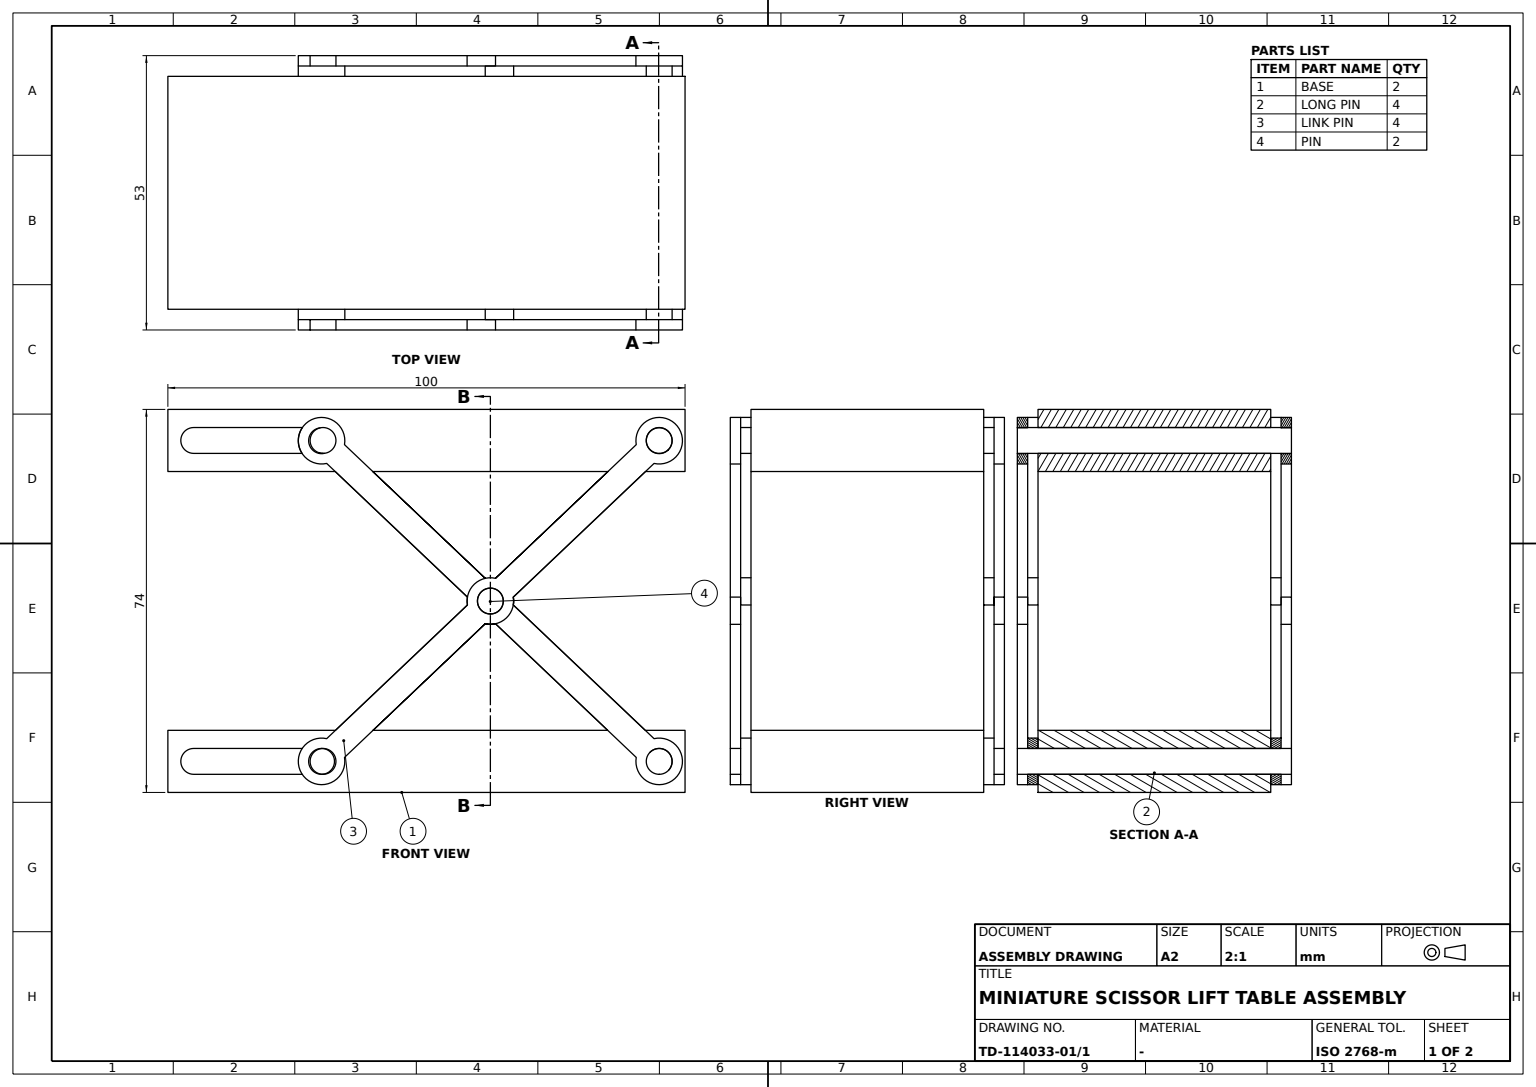
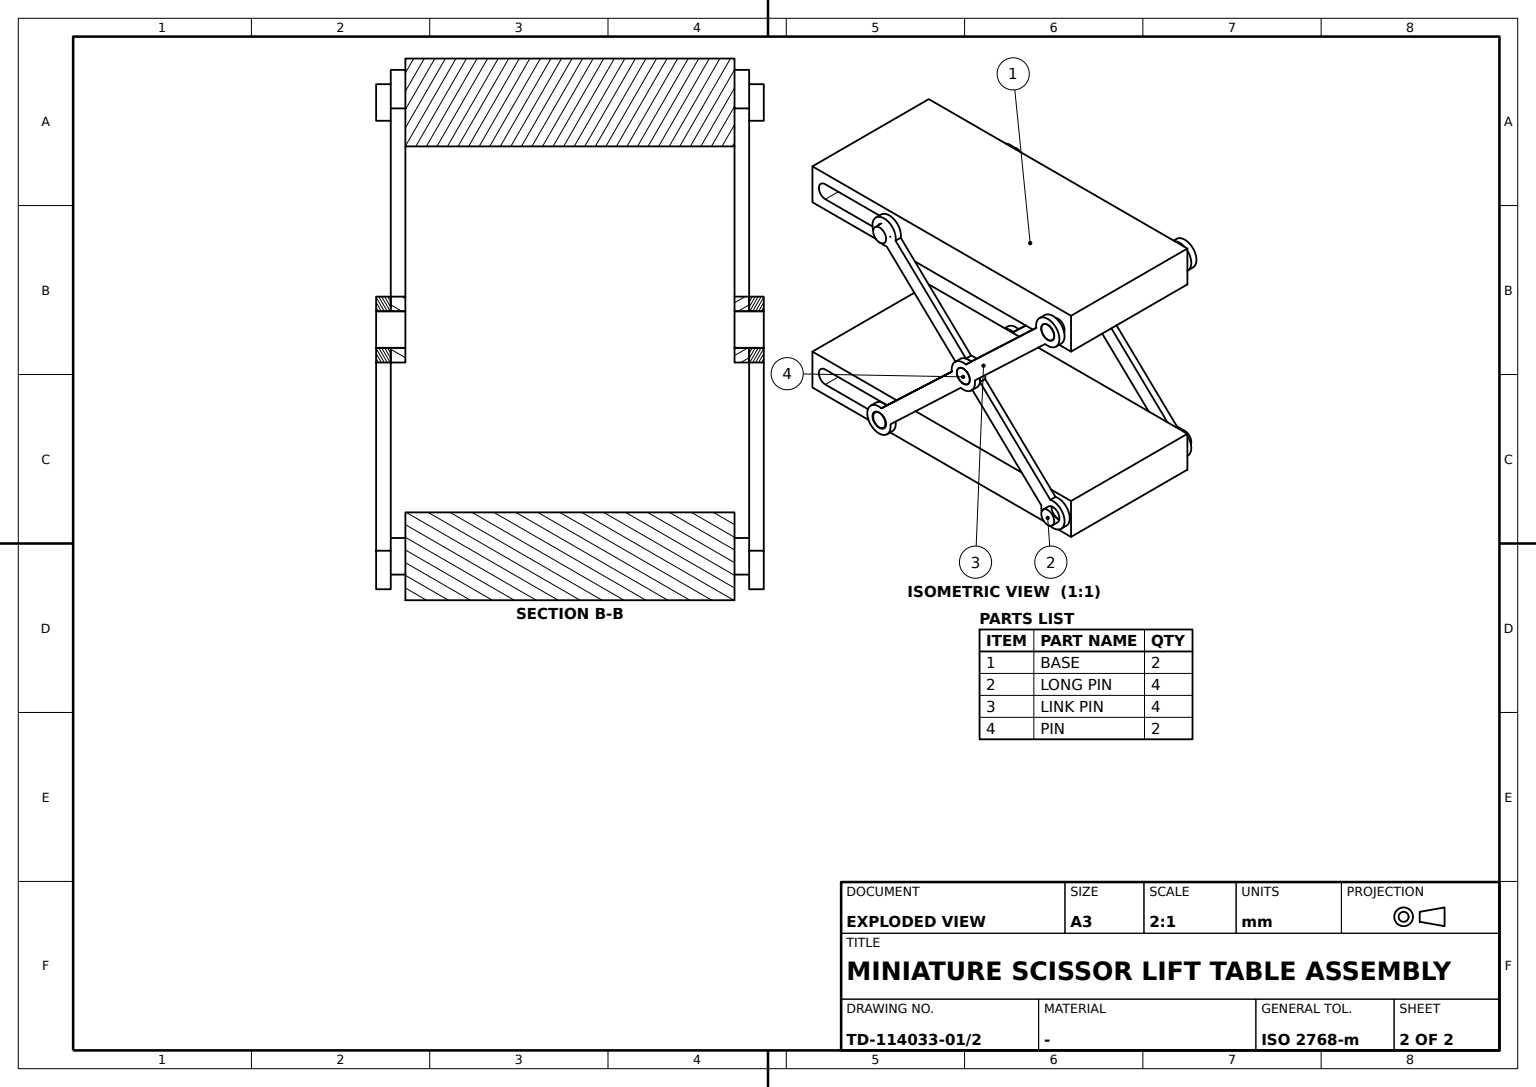
ISO-10303-21;
HEADER;
FILE_DESCRIPTION((''),'2;1');
FILE_NAME('','',(''),(''),'','','');
FILE_SCHEMA(('AUTOMOTIVE_DESIGN'));
ENDSEC;
DATA;
#11=LINE('',#845,#47);
#12=LINE('',#849,#48);
#13=LINE('',#853,#49);
#14=LINE('',#857,#50);
#15=LINE('',#865,#51);
#16=LINE('',#870,#52);
#17=LINE('',#874,#53);
#18=LINE('',#878,#54);
#19=LINE('',#885,#55);
#20=LINE('',#886,#56);
#21=LINE('',#888,#57);
#22=LINE('',#890,#58);
#23=LINE('',#892,#59);
#24=LINE('',#894,#60);
#25=LINE('',#896,#61);
#26=LINE('',#898,#62);
#27=LINE('',#917,#63);
#28=LINE('',#921,#64);
#29=LINE('',#928,#65);
#30=LINE('',#931,#66);
#31=LINE('',#933,#67);
#32=LINE('',#935,#68);
#33=LINE('',#937,#69);
#34=LINE('',#940,#70);
#35=LINE('',#941,#71);
#36=LINE('',#943,#72);
#37=LINE('',#946,#73);
#38=LINE('',#947,#74);
#39=LINE('',#949,#75);
#40=LINE('',#950,#76);
#41=LINE('',#952,#77);
#42=LINE('',#954,#78);
#43=LINE('',#956,#79);
#44=LINE('',#958,#80);
#45=LINE('',#964,#81);
#46=LINE('',#966,#82);
#47=VECTOR('',#681,1000.);
#48=VECTOR('',#684,1000.);
#49=VECTOR('',#687,1000.);
#50=VECTOR('',#690,1000.);
#51=VECTOR('',#699,1000.);
#52=VECTOR('',#702,1000.);
#53=VECTOR('',#705,1000.);
#54=VECTOR('',#708,1000.);
#55=VECTOR('',#719,1000.);
#56=VECTOR('',#720,1000.);
#57=VECTOR('',#723,1000.);
#58=VECTOR('',#726,1000.);
#59=VECTOR('',#729,1000.);
#60=VECTOR('',#732,1000.);
#61=VECTOR('',#735,1000.);
#62=VECTOR('',#738,1000.);
#63=VECTOR('',#767,1000.);
#64=VECTOR('',#770,1000.);
#65=VECTOR('',#779,1000.);
#66=VECTOR('',#780,1000.);
#67=VECTOR('',#781,1000.);
#68=VECTOR('',#782,1000.);
#69=VECTOR('',#785,1000.);
#70=VECTOR('',#786,1000.);
#71=VECTOR('',#787,1000.);
#72=VECTOR('',#790,1000.);
#73=VECTOR('',#791,1000.);
#74=VECTOR('',#792,1000.);
#75=VECTOR('',#795,1000.);
#76=VECTOR('',#796,1000.);
#77=VECTOR('',#799,1000.);
#78=VECTOR('',#800,1000.);
#79=VECTOR('',#801,1000.);
#80=VECTOR('',#804,1000.);
#81=VECTOR('',#811,1000.);
#82=VECTOR('',#814,1000.);
#83=CONTEXT_DEPENDENT_SHAPE_REPRESENTATION(#107,#988);
#84=CONTEXT_DEPENDENT_SHAPE_REPRESENTATION(#108,#989);
#85=CONTEXT_DEPENDENT_SHAPE_REPRESENTATION(#109,#991);
#86=CONTEXT_DEPENDENT_SHAPE_REPRESENTATION(#110,#992);
#87=CONTEXT_DEPENDENT_SHAPE_REPRESENTATION(#111,#993);
#88=CONTEXT_DEPENDENT_SHAPE_REPRESENTATION(#112,#994);
#89=CONTEXT_DEPENDENT_SHAPE_REPRESENTATION(#113,#996);
#90=CONTEXT_DEPENDENT_SHAPE_REPRESENTATION(#114,#997);
#91=CONTEXT_DEPENDENT_SHAPE_REPRESENTATION(#115,#999);
#92=CONTEXT_DEPENDENT_SHAPE_REPRESENTATION(#116,#1000);
#93=CONTEXT_DEPENDENT_SHAPE_REPRESENTATION(#117,#1001);
#94=CONTEXT_DEPENDENT_SHAPE_REPRESENTATION(#118,#1002);
#95=NEXT_ASSEMBLY_USAGE_OCCURRENCE('pin','pin','pin',#1003,#1004,'');
#96=NEXT_ASSEMBLY_USAGE_OCCURRENCE('pin','pin','pin',#1003,#1004,'');
#97=NEXT_ASSEMBLY_USAGE_OCCURRENCE('link pin','link pin','link pin',#1003,#1005,'');
#98=NEXT_ASSEMBLY_USAGE_OCCURRENCE('link pin','link pin','link pin',#1003,#1005,'');
#99=NEXT_ASSEMBLY_USAGE_OCCURRENCE('link pin','link pin','link pin',#1003,#1005,'');
#100=NEXT_ASSEMBLY_USAGE_OCCURRENCE('link pin','link pin','link pin',#1003,#1005,'');
#101=NEXT_ASSEMBLY_USAGE_OCCURRENCE('long pin','long pin','long pin',#1003,#1006,'');
#102=NEXT_ASSEMBLY_USAGE_OCCURRENCE('long pin','long pin','long pin',#1003,#1006,'');
#103=NEXT_ASSEMBLY_USAGE_OCCURRENCE('base','base','base',#1003,#1007,'');
#104=NEXT_ASSEMBLY_USAGE_OCCURRENCE('long pin','long pin','long pin',#1003,#1006,'');
#105=NEXT_ASSEMBLY_USAGE_OCCURRENCE('long pin','long pin','long pin',#1003,#1006,'');
#106=NEXT_ASSEMBLY_USAGE_OCCURRENCE('base','base','base',#1003,#1007,'');
#107=(REPRESENTATION_RELATIONSHIP(' ',' ',#584,#583)REPRESENTATION_RELATIONSHIP_WITH_TRANSFORMATION(#119)SHAPE_REPRESENTATION_RELATIONSHIP());
#108=(REPRESENTATION_RELATIONSHIP(' ',' ',#584,#583)REPRESENTATION_RELATIONSHIP_WITH_TRANSFORMATION(#120)SHAPE_REPRESENTATION_RELATIONSHIP());
#109=(REPRESENTATION_RELATIONSHIP(' ',' ',#585,#583)REPRESENTATION_RELATIONSHIP_WITH_TRANSFORMATION(#121)SHAPE_REPRESENTATION_RELATIONSHIP());
#110=(REPRESENTATION_RELATIONSHIP(' ',' ',#585,#583)REPRESENTATION_RELATIONSHIP_WITH_TRANSFORMATION(#122)SHAPE_REPRESENTATION_RELATIONSHIP());
#111=(REPRESENTATION_RELATIONSHIP(' ',' ',#585,#583)REPRESENTATION_RELATIONSHIP_WITH_TRANSFORMATION(#123)SHAPE_REPRESENTATION_RELATIONSHIP());
#112=(REPRESENTATION_RELATIONSHIP(' ',' ',#585,#583)REPRESENTATION_RELATIONSHIP_WITH_TRANSFORMATION(#124)SHAPE_REPRESENTATION_RELATIONSHIP());
#113=(REPRESENTATION_RELATIONSHIP(' ',' ',#586,#583)REPRESENTATION_RELATIONSHIP_WITH_TRANSFORMATION(#125)SHAPE_REPRESENTATION_RELATIONSHIP());
#114=(REPRESENTATION_RELATIONSHIP(' ',' ',#586,#583)REPRESENTATION_RELATIONSHIP_WITH_TRANSFORMATION(#126)SHAPE_REPRESENTATION_RELATIONSHIP());
#115=(REPRESENTATION_RELATIONSHIP(' ',' ',#587,#583)REPRESENTATION_RELATIONSHIP_WITH_TRANSFORMATION(#127)SHAPE_REPRESENTATION_RELATIONSHIP());
#116=(REPRESENTATION_RELATIONSHIP(' ',' ',#586,#583)REPRESENTATION_RELATIONSHIP_WITH_TRANSFORMATION(#128)SHAPE_REPRESENTATION_RELATIONSHIP());
#117=(REPRESENTATION_RELATIONSHIP(' ',' ',#586,#583)REPRESENTATION_RELATIONSHIP_WITH_TRANSFORMATION(#129)SHAPE_REPRESENTATION_RELATIONSHIP());
#118=(REPRESENTATION_RELATIONSHIP(' ',' ',#587,#583)REPRESENTATION_RELATIONSHIP_WITH_TRANSFORMATION(#130)SHAPE_REPRESENTATION_RELATIONSHIP());
#119=ITEM_DEFINED_TRANSFORMATION(' ',' ',#588,#594);
#120=ITEM_DEFINED_TRANSFORMATION(' ',' ',#588,#595);
#121=ITEM_DEFINED_TRANSFORMATION(' ',' ',#588,#623);
#122=ITEM_DEFINED_TRANSFORMATION(' ',' ',#588,#624);
#123=ITEM_DEFINED_TRANSFORMATION(' ',' ',#588,#625);
#124=ITEM_DEFINED_TRANSFORMATION(' ',' ',#588,#626);
#125=ITEM_DEFINED_TRANSFORMATION(' ',' ',#588,#632);
#126=ITEM_DEFINED_TRANSFORMATION(' ',' ',#588,#633);
#127=ITEM_DEFINED_TRANSFORMATION(' ',' ',#588,#651);
#128=ITEM_DEFINED_TRANSFORMATION(' ',' ',#588,#652);
#129=ITEM_DEFINED_TRANSFORMATION(' ',' ',#588,#653);
#130=ITEM_DEFINED_TRANSFORMATION(' ',' ',#588,#654);
#131=SHAPE_REPRESENTATION_RELATIONSHIP('','',#584,#135);
#132=SHAPE_REPRESENTATION_RELATIONSHIP('','',#585,#136);
#133=SHAPE_REPRESENTATION_RELATIONSHIP('','',#586,#137);
#134=SHAPE_REPRESENTATION_RELATIONSHIP('','',#587,#138);
#135=ADVANCED_BREP_SHAPE_REPRESENTATION('',(#574),#974);
#136=ADVANCED_BREP_SHAPE_REPRESENTATION('',(#575),#975);
#137=ADVANCED_BREP_SHAPE_REPRESENTATION('',(#576),#976);
#138=ADVANCED_BREP_SHAPE_REPRESENTATION('',(#577),#977);
#139=CYLINDRICAL_SURFACE('',#593,2.5);
#140=CYLINDRICAL_SURFACE('',#612,2.5);
#141=CYLINDRICAL_SURFACE('',#613,2.5);
#142=CYLINDRICAL_SURFACE('',#614,2.5);
#143=CYLINDRICAL_SURFACE('',#616,4.5);
#144=CYLINDRICAL_SURFACE('',#618,4.5);
#145=CYLINDRICAL_SURFACE('',#620,4.5);
#146=CYLINDRICAL_SURFACE('',#622,4.5);
#147=CYLINDRICAL_SURFACE('',#631,2.5);
#148=CYLINDRICAL_SURFACE('',#634,2.5);
#149=CYLINDRICAL_SURFACE('',#637,2.5);
#150=CYLINDRICAL_SURFACE('',#649,2.5);
#151=ORIENTED_EDGE('',*,*,#271,.T.);
#152=ORIENTED_EDGE('',*,*,#272,.F.);
#153=ORIENTED_EDGE('',*,*,#271,.F.);
#154=ORIENTED_EDGE('',*,*,#272,.T.);
#155=ORIENTED_EDGE('',*,*,#273,.F.);
#156=ORIENTED_EDGE('',*,*,#274,.F.);
#157=ORIENTED_EDGE('',*,*,#275,.F.);
#158=ORIENTED_EDGE('',*,*,#276,.T.);
#159=ORIENTED_EDGE('',*,*,#277,.T.);
#160=ORIENTED_EDGE('',*,*,#278,.T.);
#161=ORIENTED_EDGE('',*,*,#279,.T.);
#162=ORIENTED_EDGE('',*,*,#280,.T.);
#163=ORIENTED_EDGE('',*,*,#281,.F.);
#164=ORIENTED_EDGE('',*,*,#282,.T.);
#165=ORIENTED_EDGE('',*,*,#283,.F.);
#166=ORIENTED_EDGE('',*,*,#284,.T.);
#167=ORIENTED_EDGE('',*,*,#285,.T.);
#168=ORIENTED_EDGE('',*,*,#286,.T.);
#169=ORIENTED_EDGE('',*,*,#287,.T.);
#170=ORIENTED_EDGE('',*,*,#288,.F.);
#171=ORIENTED_EDGE('',*,*,#289,.T.);
#172=ORIENTED_EDGE('',*,*,#290,.F.);
#173=ORIENTED_EDGE('',*,*,#291,.F.);
#174=ORIENTED_EDGE('',*,*,#292,.F.);
#175=ORIENTED_EDGE('',*,*,#293,.F.);
#176=ORIENTED_EDGE('',*,*,#294,.F.);
#177=ORIENTED_EDGE('',*,*,#273,.T.);
#178=ORIENTED_EDGE('',*,*,#284,.F.);
#179=ORIENTED_EDGE('',*,*,#274,.T.);
#180=ORIENTED_EDGE('',*,*,#285,.F.);
#181=ORIENTED_EDGE('',*,*,#275,.T.);
#182=ORIENTED_EDGE('',*,*,#286,.F.);
#183=ORIENTED_EDGE('',*,*,#295,.F.);
#184=ORIENTED_EDGE('',*,*,#287,.F.);
#185=ORIENTED_EDGE('',*,*,#296,.T.);
#186=ORIENTED_EDGE('',*,*,#283,.T.);
#187=ORIENTED_EDGE('',*,*,#297,.F.);
#188=ORIENTED_EDGE('',*,*,#288,.T.);
#189=ORIENTED_EDGE('',*,*,#295,.T.);
#190=ORIENTED_EDGE('',*,*,#282,.F.);
#191=ORIENTED_EDGE('',*,*,#298,.F.);
#192=ORIENTED_EDGE('',*,*,#289,.F.);
#193=ORIENTED_EDGE('',*,*,#297,.T.);
#194=ORIENTED_EDGE('',*,*,#281,.T.);
#195=ORIENTED_EDGE('',*,*,#299,.F.);
#196=ORIENTED_EDGE('',*,*,#290,.T.);
#197=ORIENTED_EDGE('',*,*,#298,.T.);
#198=ORIENTED_EDGE('',*,*,#280,.F.);
#199=ORIENTED_EDGE('',*,*,#300,.F.);
#200=ORIENTED_EDGE('',*,*,#291,.T.);
#201=ORIENTED_EDGE('',*,*,#299,.T.);
#202=ORIENTED_EDGE('',*,*,#279,.F.);
#203=ORIENTED_EDGE('',*,*,#301,.F.);
#204=ORIENTED_EDGE('',*,*,#292,.T.);
#205=ORIENTED_EDGE('',*,*,#300,.T.);
#206=ORIENTED_EDGE('',*,*,#278,.F.);
#207=ORIENTED_EDGE('',*,*,#302,.F.);
#208=ORIENTED_EDGE('',*,*,#293,.T.);
#209=ORIENTED_EDGE('',*,*,#301,.T.);
#210=ORIENTED_EDGE('',*,*,#277,.F.);
#211=ORIENTED_EDGE('',*,*,#296,.F.);
#212=ORIENTED_EDGE('',*,*,#294,.T.);
#213=ORIENTED_EDGE('',*,*,#302,.T.);
#214=ORIENTED_EDGE('',*,*,#276,.F.);
#215=ORIENTED_EDGE('',*,*,#303,.T.);
#216=ORIENTED_EDGE('',*,*,#304,.F.);
#217=ORIENTED_EDGE('',*,*,#303,.F.);
#218=ORIENTED_EDGE('',*,*,#304,.T.);
#219=ORIENTED_EDGE('',*,*,#305,.F.);
#220=ORIENTED_EDGE('',*,*,#306,.F.);
#221=ORIENTED_EDGE('',*,*,#307,.T.);
#222=ORIENTED_EDGE('',*,*,#308,.T.);
#223=ORIENTED_EDGE('',*,*,#309,.F.);
#224=ORIENTED_EDGE('',*,*,#310,.T.);
#225=ORIENTED_EDGE('',*,*,#311,.F.);
#226=ORIENTED_EDGE('',*,*,#312,.F.);
#227=ORIENTED_EDGE('',*,*,#313,.T.);
#228=ORIENTED_EDGE('',*,*,#314,.T.);
#229=ORIENTED_EDGE('',*,*,#315,.F.);
#230=ORIENTED_EDGE('',*,*,#316,.F.);
#231=ORIENTED_EDGE('',*,*,#311,.T.);
#232=ORIENTED_EDGE('',*,*,#317,.T.);
#233=ORIENTED_EDGE('',*,*,#318,.F.);
#234=ORIENTED_EDGE('',*,*,#319,.F.);
#235=ORIENTED_EDGE('',*,*,#315,.T.);
#236=ORIENTED_EDGE('',*,*,#320,.T.);
#237=ORIENTED_EDGE('',*,*,#313,.F.);
#238=ORIENTED_EDGE('',*,*,#321,.F.);
#239=ORIENTED_EDGE('',*,*,#318,.T.);
#240=ORIENTED_EDGE('',*,*,#322,.T.);
#241=ORIENTED_EDGE('',*,*,#323,.T.);
#242=ORIENTED_EDGE('',*,*,#324,.F.);
#243=ORIENTED_EDGE('',*,*,#325,.F.);
#244=ORIENTED_EDGE('',*,*,#306,.T.);
#245=ORIENTED_EDGE('',*,*,#309,.T.);
#246=ORIENTED_EDGE('',*,*,#326,.F.);
#247=ORIENTED_EDGE('',*,*,#327,.T.);
#248=ORIENTED_EDGE('',*,*,#323,.F.);
#249=ORIENTED_EDGE('',*,*,#305,.T.);
#250=ORIENTED_EDGE('',*,*,#312,.T.);
#251=ORIENTED_EDGE('',*,*,#316,.T.);
#252=ORIENTED_EDGE('',*,*,#319,.T.);
#253=ORIENTED_EDGE('',*,*,#321,.T.);
#254=ORIENTED_EDGE('',*,*,#310,.F.);
#255=ORIENTED_EDGE('',*,*,#307,.F.);
#256=ORIENTED_EDGE('',*,*,#325,.T.);
#257=ORIENTED_EDGE('',*,*,#328,.F.);
#258=ORIENTED_EDGE('',*,*,#329,.T.);
#259=ORIENTED_EDGE('',*,*,#322,.F.);
#260=ORIENTED_EDGE('',*,*,#320,.F.);
#261=ORIENTED_EDGE('',*,*,#317,.F.);
#262=ORIENTED_EDGE('',*,*,#314,.F.);
#263=ORIENTED_EDGE('',*,*,#327,.F.);
#264=ORIENTED_EDGE('',*,*,#330,.F.);
#265=ORIENTED_EDGE('',*,*,#328,.T.);
#266=ORIENTED_EDGE('',*,*,#324,.T.);
#267=ORIENTED_EDGE('',*,*,#326,.T.);
#268=ORIENTED_EDGE('',*,*,#308,.F.);
#269=ORIENTED_EDGE('',*,*,#329,.F.);
#270=ORIENTED_EDGE('',*,*,#330,.T.);
#271=EDGE_CURVE('',#331,#331,#375,.T.);
#272=EDGE_CURVE('',#332,#332,#376,.T.);
#273=EDGE_CURVE('',#333,#333,#377,.T.);
#274=EDGE_CURVE('',#334,#334,#378,.T.);
#275=EDGE_CURVE('',#335,#335,#379,.T.);
#276=EDGE_CURVE('',#336,#337,#380,.T.);
#277=EDGE_CURVE('',#337,#338,#11,.T.);
#278=EDGE_CURVE('',#338,#339,#381,.T.);
#279=EDGE_CURVE('',#339,#340,#12,.T.);
#280=EDGE_CURVE('',#340,#341,#382,.T.);
#281=EDGE_CURVE('',#342,#341,#13,.T.);
#282=EDGE_CURVE('',#342,#343,#383,.T.);
#283=EDGE_CURVE('',#336,#343,#14,.T.);
#284=EDGE_CURVE('',#344,#344,#384,.T.);
#285=EDGE_CURVE('',#345,#345,#385,.T.);
#286=EDGE_CURVE('',#346,#346,#386,.T.);
#287=EDGE_CURVE('',#347,#348,#15,.T.);
#288=EDGE_CURVE('',#349,#348,#387,.T.);
#289=EDGE_CURVE('',#349,#350,#16,.T.);
#290=EDGE_CURVE('',#351,#350,#388,.T.);
#291=EDGE_CURVE('',#352,#351,#17,.T.);
#292=EDGE_CURVE('',#353,#352,#389,.T.);
#293=EDGE_CURVE('',#354,#353,#18,.T.);
#294=EDGE_CURVE('',#347,#354,#390,.T.);
#295=EDGE_CURVE('',#348,#343,#19,.T.);
#296=EDGE_CURVE('',#347,#336,#20,.T.);
#297=EDGE_CURVE('',#349,#342,#21,.T.);
#298=EDGE_CURVE('',#350,#341,#22,.T.);
#299=EDGE_CURVE('',#351,#340,#23,.T.);
#300=EDGE_CURVE('',#352,#339,#24,.T.);
#301=EDGE_CURVE('',#353,#338,#25,.T.);
#302=EDGE_CURVE('',#354,#337,#26,.T.);
#303=EDGE_CURVE('',#355,#355,#391,.T.);
#304=EDGE_CURVE('',#356,#356,#392,.T.);
#305=EDGE_CURVE('',#357,#358,#393,.T.);
#306=EDGE_CURVE('',#359,#357,#27,.F.);
#307=EDGE_CURVE('',#359,#360,#394,.T.);
#308=EDGE_CURVE('',#360,#358,#28,.F.);
#309=EDGE_CURVE('',#361,#361,#395,.T.);
#310=EDGE_CURVE('',#362,#362,#396,.T.);
#311=EDGE_CURVE('',#363,#364,#29,.T.);
#312=EDGE_CURVE('',#365,#363,#30,.T.);
#313=EDGE_CURVE('',#365,#366,#31,.T.);
#314=EDGE_CURVE('',#366,#364,#32,.T.);
#315=EDGE_CURVE('',#367,#368,#33,.T.);
#316=EDGE_CURVE('',#363,#367,#34,.T.);
#317=EDGE_CURVE('',#364,#368,#35,.T.);
#318=EDGE_CURVE('',#369,#370,#36,.T.);
#319=EDGE_CURVE('',#367,#369,#37,.T.);
#320=EDGE_CURVE('',#368,#370,#38,.T.);
#321=EDGE_CURVE('',#369,#365,#39,.T.);
#322=EDGE_CURVE('',#370,#366,#40,.T.);
#323=EDGE_CURVE('',#357,#371,#41,.T.);
#324=EDGE_CURVE('',#372,#371,#42,.F.);
#325=EDGE_CURVE('',#359,#372,#43,.T.);
#326=EDGE_CURVE('',#373,#358,#44,.T.);
#327=EDGE_CURVE('',#373,#371,#397,.T.);
#328=EDGE_CURVE('',#374,#372,#398,.T.);
#329=EDGE_CURVE('',#374,#360,#45,.T.);
#330=EDGE_CURVE('',#374,#373,#46,.F.);
#331=VERTEX_POINT('',#828);
#332=VERTEX_POINT('',#831);
#333=VERTEX_POINT('',#837);
#334=VERTEX_POINT('',#839);
#335=VERTEX_POINT('',#841);
#336=VERTEX_POINT('',#843);
#337=VERTEX_POINT('',#844);
#338=VERTEX_POINT('',#846);
#339=VERTEX_POINT('',#848);
#340=VERTEX_POINT('',#850);
#341=VERTEX_POINT('',#852);
#342=VERTEX_POINT('',#854);
#343=VERTEX_POINT('',#856);
#344=VERTEX_POINT('',#860);
#345=VERTEX_POINT('',#862);
#346=VERTEX_POINT('',#864);
#347=VERTEX_POINT('',#866);
#348=VERTEX_POINT('',#867);
#349=VERTEX_POINT('',#869);
#350=VERTEX_POINT('',#871);
#351=VERTEX_POINT('',#873);
#352=VERTEX_POINT('',#875);
#353=VERTEX_POINT('',#877);
#354=VERTEX_POINT('',#879);
#355=VERTEX_POINT('',#906);
#356=VERTEX_POINT('',#909);
#357=VERTEX_POINT('',#915);
#358=VERTEX_POINT('',#916);
#359=VERTEX_POINT('',#918);
#360=VERTEX_POINT('',#920);
#361=VERTEX_POINT('',#924);
#362=VERTEX_POINT('',#926);
#363=VERTEX_POINT('',#929);
#364=VERTEX_POINT('',#930);
#365=VERTEX_POINT('',#932);
#366=VERTEX_POINT('',#934);
#367=VERTEX_POINT('',#938);
#368=VERTEX_POINT('',#939);
#369=VERTEX_POINT('',#944);
#370=VERTEX_POINT('',#945);
#371=VERTEX_POINT('',#953);
#372=VERTEX_POINT('',#955);
#373=VERTEX_POINT('',#959);
#374=VERTEX_POINT('',#963);
#375=CIRCLE('',#590,2.5);
#376=CIRCLE('',#592,2.5);
#377=CIRCLE('',#597,2.5);
#378=CIRCLE('',#598,2.5);
#379=CIRCLE('',#599,2.5);
#380=CIRCLE('',#600,4.5);
#381=CIRCLE('',#601,4.5);
#382=CIRCLE('',#602,4.5);
#383=CIRCLE('',#603,4.5);
#384=CIRCLE('',#605,2.5);
#385=CIRCLE('',#606,2.5);
#386=CIRCLE('',#607,2.5);
#387=CIRCLE('',#608,4.5);
#388=CIRCLE('',#609,4.5);
#389=CIRCLE('',#610,4.5);
#390=CIRCLE('',#611,4.5);
#391=CIRCLE('',#628,2.5);
#392=CIRCLE('',#630,2.5);
#393=CIRCLE('',#635,2.5);
#394=CIRCLE('',#636,2.5);
#395=CIRCLE('',#638,2.5);
#396=CIRCLE('',#639,2.5);
#397=CIRCLE('',#646,2.5);
#398=CIRCLE('',#648,2.5);
#399=EDGE_LOOP('',(#151));
#400=EDGE_LOOP('',(#152));
#401=EDGE_LOOP('',(#153));
#402=EDGE_LOOP('',(#154));
#403=EDGE_LOOP('',(#155));
#404=EDGE_LOOP('',(#156));
#405=EDGE_LOOP('',(#157));
#406=EDGE_LOOP('',(#158,#159,#160,#161,#162,#163,#164,#165));
#407=EDGE_LOOP('',(#166));
#408=EDGE_LOOP('',(#167));
#409=EDGE_LOOP('',(#168));
#410=EDGE_LOOP('',(#169,#170,#171,#172,#173,#174,#175,#176));
#411=EDGE_LOOP('',(#177));
#412=EDGE_LOOP('',(#178));
#413=EDGE_LOOP('',(#179));
#414=EDGE_LOOP('',(#180));
#415=EDGE_LOOP('',(#181));
#416=EDGE_LOOP('',(#182));
#417=EDGE_LOOP('',(#183,#184,#185,#186));
#418=EDGE_LOOP('',(#187,#188,#189,#190));
#419=EDGE_LOOP('',(#191,#192,#193,#194));
#420=EDGE_LOOP('',(#195,#196,#197,#198));
#421=EDGE_LOOP('',(#199,#200,#201,#202));
#422=EDGE_LOOP('',(#203,#204,#205,#206));
#423=EDGE_LOOP('',(#207,#208,#209,#210));
#424=EDGE_LOOP('',(#211,#212,#213,#214));
#425=EDGE_LOOP('',(#215));
#426=EDGE_LOOP('',(#216));
#427=EDGE_LOOP('',(#217));
#428=EDGE_LOOP('',(#218));
#429=EDGE_LOOP('',(#219,#220,#221,#222));
#430=EDGE_LOOP('',(#223));
#431=EDGE_LOOP('',(#224));
#432=EDGE_LOOP('',(#225,#226,#227,#228));
#433=EDGE_LOOP('',(#229,#230,#231,#232));
#434=EDGE_LOOP('',(#233,#234,#235,#236));
#435=EDGE_LOOP('',(#237,#238,#239,#240));
#436=EDGE_LOOP('',(#241,#242,#243,#244));
#437=EDGE_LOOP('',(#245));
#438=EDGE_LOOP('',(#246,#247,#248,#249));
#439=EDGE_LOOP('',(#250,#251,#252,#253));
#440=EDGE_LOOP('',(#254));
#441=EDGE_LOOP('',(#255,#256,#257,#258));
#442=EDGE_LOOP('',(#259,#260,#261,#262));
#443=EDGE_LOOP('',(#263,#264,#265,#266));
#444=EDGE_LOOP('',(#267,#268,#269,#270));
#445=FACE_BOUND('',#399,.T.);
#446=FACE_BOUND('',#400,.T.);
#447=FACE_BOUND('',#401,.T.);
#448=FACE_BOUND('',#402,.T.);
#449=FACE_BOUND('',#403,.T.);
#450=FACE_BOUND('',#404,.T.);
#451=FACE_BOUND('',#405,.T.);
#452=FACE_BOUND('',#406,.T.);
#453=FACE_BOUND('',#407,.T.);
#454=FACE_BOUND('',#408,.T.);
#455=FACE_BOUND('',#409,.T.);
#456=FACE_BOUND('',#410,.T.);
#457=FACE_BOUND('',#411,.T.);
#458=FACE_BOUND('',#412,.T.);
#459=FACE_BOUND('',#413,.T.);
#460=FACE_BOUND('',#414,.T.);
#461=FACE_BOUND('',#415,.T.);
#462=FACE_BOUND('',#416,.T.);
#463=FACE_BOUND('',#417,.T.);
#464=FACE_BOUND('',#418,.T.);
#465=FACE_BOUND('',#419,.T.);
#466=FACE_BOUND('',#420,.T.);
#467=FACE_BOUND('',#421,.T.);
#468=FACE_BOUND('',#422,.T.);
#469=FACE_BOUND('',#423,.T.);
#470=FACE_BOUND('',#424,.T.);
#471=FACE_BOUND('',#425,.T.);
#472=FACE_BOUND('',#426,.T.);
#473=FACE_BOUND('',#427,.T.);
#474=FACE_BOUND('',#428,.T.);
#475=FACE_BOUND('',#429,.T.);
#476=FACE_BOUND('',#430,.T.);
#477=FACE_BOUND('',#431,.T.);
#478=FACE_BOUND('',#432,.T.);
#479=FACE_BOUND('',#433,.T.);
#480=FACE_BOUND('',#434,.T.);
#481=FACE_BOUND('',#435,.T.);
#482=FACE_BOUND('',#436,.T.);
#483=FACE_BOUND('',#437,.T.);
#484=FACE_BOUND('',#438,.T.);
#485=FACE_BOUND('',#439,.T.);
#486=FACE_BOUND('',#440,.T.);
#487=FACE_BOUND('',#441,.T.);
#488=FACE_BOUND('',#442,.T.);
#489=FACE_BOUND('',#443,.T.);
#490=FACE_BOUND('',#444,.T.);
#491=PLANE('',#589);
#492=PLANE('',#591);
#493=PLANE('',#596);
#494=PLANE('',#604);
#495=PLANE('',#615);
#496=PLANE('',#617);
#497=PLANE('',#619);
#498=PLANE('',#621);
#499=PLANE('',#627);
#500=PLANE('',#629);
#501=PLANE('',#640);
#502=PLANE('',#641);
#503=PLANE('',#642);
#504=PLANE('',#643);
#505=PLANE('',#644);
#506=PLANE('',#645);
#507=PLANE('',#647);
#508=PLANE('',#650);
#509=ADVANCED_FACE('',(#445),#491,.T.);
#510=ADVANCED_FACE('',(#446),#492,.F.);
#511=ADVANCED_FACE('',(#447,#448),#139,.T.);
#512=ADVANCED_FACE('',(#449,#450,#451,#452),#493,.T.);
#513=ADVANCED_FACE('',(#453,#454,#455,#456),#494,.F.);
#514=ADVANCED_FACE('',(#457,#458),#140,.F.);
#515=ADVANCED_FACE('',(#459,#460),#141,.F.);
#516=ADVANCED_FACE('',(#461,#462),#142,.F.);
#517=ADVANCED_FACE('',(#463),#495,.F.);
#518=ADVANCED_FACE('',(#464),#143,.T.);
#519=ADVANCED_FACE('',(#465),#496,.F.);
#520=ADVANCED_FACE('',(#466),#144,.T.);
#521=ADVANCED_FACE('',(#467),#497,.T.);
#522=ADVANCED_FACE('',(#468),#145,.T.);
#523=ADVANCED_FACE('',(#469),#498,.T.);
#524=ADVANCED_FACE('',(#470),#146,.T.);
#525=ADVANCED_FACE('',(#471),#499,.T.);
#526=ADVANCED_FACE('',(#472),#500,.F.);
#527=ADVANCED_FACE('',(#473,#474),#147,.T.);
#528=ADVANCED_FACE('',(#475),#148,.F.);
#529=ADVANCED_FACE('',(#476,#477),#149,.F.);
#530=ADVANCED_FACE('',(#478),#501,.F.);
#531=ADVANCED_FACE('',(#479),#502,.F.);
#532=ADVANCED_FACE('',(#480),#503,.F.);
#533=ADVANCED_FACE('',(#481),#504,.F.);
#534=ADVANCED_FACE('',(#482),#505,.F.);
#535=ADVANCED_FACE('',(#483,#484,#485),#506,.F.);
#536=ADVANCED_FACE('',(#486,#487,#488),#507,.T.);
#537=ADVANCED_FACE('',(#489),#150,.F.);
#538=ADVANCED_FACE('',(#490),#508,.F.);
#539=CLOSED_SHELL('',(#509,#510,#511));
#540=CLOSED_SHELL('',(#512,#513,#514,#515,#516,#517,#518,#519,#520,#521,#522,#523,#524));
#541=CLOSED_SHELL('',(#525,#526,#527));
#542=CLOSED_SHELL('',(#528,#529,#530,#531,#532,#533,#534,#535,#536,#537,#538));
#574=MANIFOLD_SOLID_BREP('',#539);
#575=MANIFOLD_SOLID_BREP('',#540);
#576=MANIFOLD_SOLID_BREP('',#541);
#577=MANIFOLD_SOLID_BREP('',#542);
#578=SHAPE_DEFINITION_REPRESENTATION(#986,#583);
#579=SHAPE_DEFINITION_REPRESENTATION(#987,#584);
#580=SHAPE_DEFINITION_REPRESENTATION(#990,#585);
#581=SHAPE_DEFINITION_REPRESENTATION(#995,#586);
#582=SHAPE_DEFINITION_REPRESENTATION(#998,#587);
#583=SHAPE_REPRESENTATION('',(#588,#594,#595,#623,#624,#625,#626,#632,#633,#651,#652,#653,#654),#973);
#584=SHAPE_REPRESENTATION('',(#588),#974);
#585=SHAPE_REPRESENTATION('',(#588),#975);
#586=SHAPE_REPRESENTATION('',(#588),#976);
#587=SHAPE_REPRESENTATION('',(#588),#977);
#588=AXIS2_PLACEMENT_3D('',#825,#655,#656);
#589=AXIS2_PLACEMENT_3D('',#826,#657,#658);
#590=AXIS2_PLACEMENT_3D('',#827,#659,#660);
#591=AXIS2_PLACEMENT_3D('',#829,#661,#662);
#592=AXIS2_PLACEMENT_3D('',#830,#663,#664);
#593=AXIS2_PLACEMENT_3D('',#832,#665,#666);
#594=AXIS2_PLACEMENT_3D('',#833,#667,#668);
#595=AXIS2_PLACEMENT_3D('',#834,#669,#670);
#596=AXIS2_PLACEMENT_3D('',#835,#671,#672);
#597=AXIS2_PLACEMENT_3D('',#836,#673,#674);
#598=AXIS2_PLACEMENT_3D('',#838,#675,#676);
#599=AXIS2_PLACEMENT_3D('',#840,#677,#678);
#600=AXIS2_PLACEMENT_3D('',#842,#679,#680);
#601=AXIS2_PLACEMENT_3D('',#847,#682,#683);
#602=AXIS2_PLACEMENT_3D('',#851,#685,#686);
#603=AXIS2_PLACEMENT_3D('',#855,#688,#689);
#604=AXIS2_PLACEMENT_3D('',#858,#691,#692);
#605=AXIS2_PLACEMENT_3D('',#859,#693,#694);
#606=AXIS2_PLACEMENT_3D('',#861,#695,#696);
#607=AXIS2_PLACEMENT_3D('',#863,#697,#698);
#608=AXIS2_PLACEMENT_3D('',#868,#700,#701);
#609=AXIS2_PLACEMENT_3D('',#872,#703,#704);
#610=AXIS2_PLACEMENT_3D('',#876,#706,#707);
#611=AXIS2_PLACEMENT_3D('',#880,#709,#710);
#612=AXIS2_PLACEMENT_3D('',#881,#711,#712);
#613=AXIS2_PLACEMENT_3D('',#882,#713,#714);
#614=AXIS2_PLACEMENT_3D('',#883,#715,#716);
#615=AXIS2_PLACEMENT_3D('',#884,#717,#718);
#616=AXIS2_PLACEMENT_3D('',#887,#721,#722);
#617=AXIS2_PLACEMENT_3D('',#889,#724,#725);
#618=AXIS2_PLACEMENT_3D('',#891,#727,#728);
#619=AXIS2_PLACEMENT_3D('',#893,#730,#731);
#620=AXIS2_PLACEMENT_3D('',#895,#733,#734);
#621=AXIS2_PLACEMENT_3D('',#897,#736,#737);
#622=AXIS2_PLACEMENT_3D('',#899,#739,#740);
#623=AXIS2_PLACEMENT_3D('',#900,#741,#742);
#624=AXIS2_PLACEMENT_3D('',#901,#743,#744);
#625=AXIS2_PLACEMENT_3D('',#902,#745,#746);
#626=AXIS2_PLACEMENT_3D('',#903,#747,#748);
#627=AXIS2_PLACEMENT_3D('',#904,#749,#750);
#628=AXIS2_PLACEMENT_3D('',#905,#751,#752);
#629=AXIS2_PLACEMENT_3D('',#907,#753,#754);
#630=AXIS2_PLACEMENT_3D('',#908,#755,#756);
#631=AXIS2_PLACEMENT_3D('',#910,#757,#758);
#632=AXIS2_PLACEMENT_3D('',#911,#759,#760);
#633=AXIS2_PLACEMENT_3D('',#912,#761,#762);
#634=AXIS2_PLACEMENT_3D('',#913,#763,#764);
#635=AXIS2_PLACEMENT_3D('',#914,#765,#766);
#636=AXIS2_PLACEMENT_3D('',#919,#768,#769);
#637=AXIS2_PLACEMENT_3D('',#922,#771,#772);
#638=AXIS2_PLACEMENT_3D('',#923,#773,#774);
#639=AXIS2_PLACEMENT_3D('',#925,#775,#776);
#640=AXIS2_PLACEMENT_3D('',#927,#777,#778);
#641=AXIS2_PLACEMENT_3D('',#936,#783,#784);
#642=AXIS2_PLACEMENT_3D('',#942,#788,#789);
#643=AXIS2_PLACEMENT_3D('',#948,#793,#794);
#644=AXIS2_PLACEMENT_3D('',#951,#797,#798);
#645=AXIS2_PLACEMENT_3D('',#957,#802,#803);
#646=AXIS2_PLACEMENT_3D('',#960,#805,#806);
#647=AXIS2_PLACEMENT_3D('',#961,#807,#808);
#648=AXIS2_PLACEMENT_3D('',#962,#809,#810);
#649=AXIS2_PLACEMENT_3D('',#965,#812,#813);
#650=AXIS2_PLACEMENT_3D('',#967,#815,#816);
#651=AXIS2_PLACEMENT_3D('',#968,#817,#818);
#652=AXIS2_PLACEMENT_3D('',#969,#819,#820);
#653=AXIS2_PLACEMENT_3D('',#970,#821,#822);
#654=AXIS2_PLACEMENT_3D('',#971,#823,#824);
#655=DIRECTION('',(0.,0.,1.));
#656=DIRECTION('',(1.,0.,0.));
#657=DIRECTION('',(1.,0.,0.));
#658=DIRECTION('',(0.,1.,0.));
#659=DIRECTION('',(1.,0.,0.));
#660=DIRECTION('',(0.,0.,-1.));
#661=DIRECTION('',(1.,0.,0.));
#662=DIRECTION('',(0.,1.,0.));
#663=DIRECTION('',(1.,0.,0.));
#664=DIRECTION('',(0.,0.,-1.));
#665=DIRECTION('',(1.,0.,0.));
#666=DIRECTION('',(0.,1.,0.));
#667=DIRECTION('',(0.,0.,1.));
#668=DIRECTION('',(1.,0.,0.));
#669=DIRECTION('',(0.,0.,1.));
#670=DIRECTION('',(1.,0.,0.));
#671=DIRECTION('',(1.,0.,0.));
#672=DIRECTION('',(0.,1.,0.));
#673=DIRECTION('',(1.,0.,0.));
#674=DIRECTION('',(0.,0.,-1.));
#675=DIRECTION('',(1.,0.,0.));
#676=DIRECTION('',(0.,0.,-1.));
#677=DIRECTION('',(1.,0.,0.));
#678=DIRECTION('',(0.,0.,-1.));
#679=DIRECTION('',(1.,0.,0.));
#680=DIRECTION('',(0.,0.,-1.));
#681=DIRECTION('',(0.,1.,0.));
#682=DIRECTION('',(1.,0.,0.));
#683=DIRECTION('',(0.,0.,-1.));
#684=DIRECTION('',(0.,1.,0.));
#685=DIRECTION('',(1.,0.,0.));
#686=DIRECTION('',(0.,0.,-1.));
#687=DIRECTION('',(0.,1.,0.));
#688=DIRECTION('',(1.,0.,0.));
#689=DIRECTION('',(0.,0.,-1.));
#690=DIRECTION('',(0.,1.,0.));
#691=DIRECTION('',(1.,0.,0.));
#692=DIRECTION('',(0.,1.,0.));
#693=DIRECTION('',(1.,0.,0.));
#694=DIRECTION('',(0.,0.,-1.));
#695=DIRECTION('',(1.,0.,0.));
#696=DIRECTION('',(0.,0.,-1.));
#697=DIRECTION('',(1.,0.,0.));
#698=DIRECTION('',(0.,0.,-1.));
#699=DIRECTION('',(0.,1.,0.));
#700=DIRECTION('',(1.,0.,0.));
#701=DIRECTION('',(0.,0.,-1.));
#702=DIRECTION('',(0.,1.,0.));
#703=DIRECTION('',(1.,0.,0.));
#704=DIRECTION('',(0.,0.,-1.));
#705=DIRECTION('',(0.,1.,0.));
#706=DIRECTION('',(1.,0.,0.));
#707=DIRECTION('',(0.,0.,-1.));
#708=DIRECTION('',(0.,1.,0.));
#709=DIRECTION('',(1.,0.,0.));
#710=DIRECTION('',(0.,0.,-1.));
#711=DIRECTION('',(1.,0.,0.));
#712=DIRECTION('',(0.,1.,0.));
#713=DIRECTION('',(1.,0.,0.));
#714=DIRECTION('',(0.,1.,0.));
#715=DIRECTION('',(1.,0.,0.));
#716=DIRECTION('',(0.,1.,0.));
#717=DIRECTION('',(0.,0.,-1.));
#718=DIRECTION('',(0.,1.,0.));
#719=DIRECTION('',(1.,0.,0.));
#720=DIRECTION('',(1.,0.,0.));
#721=DIRECTION('',(1.,0.,0.));
#722=DIRECTION('',(0.,1.,0.));
#723=DIRECTION('',(1.,0.,0.));
#724=DIRECTION('',(0.,0.,-1.));
#725=DIRECTION('',(0.,1.,0.));
#726=DIRECTION('',(1.,0.,0.));
#727=DIRECTION('',(1.,0.,0.));
#728=DIRECTION('',(0.,1.,0.));
#729=DIRECTION('',(1.,0.,0.));
#730=DIRECTION('',(0.,0.,-1.));
#731=DIRECTION('',(0.,1.,0.));
#732=DIRECTION('',(1.,0.,0.));
#733=DIRECTION('',(1.,0.,0.));
#734=DIRECTION('',(0.,1.,0.));
#735=DIRECTION('',(1.,0.,0.));
#736=DIRECTION('',(0.,0.,-1.));
#737=DIRECTION('',(0.,1.,0.));
#738=DIRECTION('',(1.,0.,0.));
#739=DIRECTION('',(1.,0.,0.));
#740=DIRECTION('',(0.,1.,0.));
#741=DIRECTION('',(0.,-0.688354548336075,0.725374396973754));
#742=DIRECTION('',(1.,0.,0.));
#743=DIRECTION('',(0.,-0.688354548336075,0.725374396973754));
#744=DIRECTION('',(1.,0.,0.));
#745=DIRECTION('',(0.,0.688354548336075,0.725374396973754));
#746=DIRECTION('',(1.,0.,0.));
#747=DIRECTION('',(0.,0.688354548336075,0.725374396973754));
#748=DIRECTION('',(1.,0.,0.));
#749=DIRECTION('',(1.,0.,0.));
#750=DIRECTION('',(0.,1.,0.));
#751=DIRECTION('',(1.,0.,0.));
#752=DIRECTION('',(0.,0.,-1.));
#753=DIRECTION('',(1.,0.,0.));
#754=DIRECTION('',(0.,1.,0.));
#755=DIRECTION('',(1.,0.,0.));
#756=DIRECTION('',(0.,0.,-1.));
#757=DIRECTION('',(1.,0.,0.));
#758=DIRECTION('',(0.,1.,0.));
#759=DIRECTION('',(0.,0.,1.));
#760=DIRECTION('',(1.,0.,0.));
#761=DIRECTION('',(0.,0.,1.));
#762=DIRECTION('',(1.,0.,0.));
#763=DIRECTION('',(1.,0.,0.));
#764=DIRECTION('',(0.,1.,0.));
#765=DIRECTION('',(1.,0.,0.));
#766=DIRECTION('',(0.,0.,-1.));
#767=DIRECTION('',(1.,0.,0.));
#768=DIRECTION('',(1.,0.,0.));
#769=DIRECTION('',(0.,0.,-1.));
#770=DIRECTION('',(1.,0.,0.));
#771=DIRECTION('',(1.,0.,0.));
#772=DIRECTION('',(0.,1.,0.));
#773=DIRECTION('',(1.,0.,0.));
#774=DIRECTION('',(0.,0.,-1.));
#775=DIRECTION('',(1.,0.,0.));
#776=DIRECTION('',(0.,0.,-1.));
#777=DIRECTION('',(0.,-1.,0.));
#778=DIRECTION('',(0.,0.,-1.));
#779=DIRECTION('',(1.,0.,0.));
#780=DIRECTION('',(0.,0.,-1.));
#781=DIRECTION('',(1.,0.,0.));
#782=DIRECTION('',(0.,0.,-1.));
#783=DIRECTION('',(0.,0.,1.));
#784=DIRECTION('',(0.,-1.,0.));
#785=DIRECTION('',(1.,0.,0.));
#786=DIRECTION('',(0.,-1.,0.));
#787=DIRECTION('',(0.,-1.,0.));
#788=DIRECTION('',(0.,1.,0.));
#789=DIRECTION('',(0.,0.,1.));
#790=DIRECTION('',(1.,0.,0.));
#791=DIRECTION('',(0.,0.,1.));
#792=DIRECTION('',(0.,0.,1.));
#793=DIRECTION('',(0.,0.,-1.));
#794=DIRECTION('',(0.,1.,0.));
#795=DIRECTION('',(0.,1.,0.));
#796=DIRECTION('',(0.,1.,0.));
#797=DIRECTION('',(0.,0.,-1.));
#798=DIRECTION('',(0.,-1.,0.));
#799=DIRECTION('',(0.,-1.,0.));
#800=DIRECTION('',(1.,0.,0.));
#801=DIRECTION('',(0.,-1.,0.));
#802=DIRECTION('',(1.,0.,0.));
#803=DIRECTION('',(0.,1.,0.));
#804=DIRECTION('',(0.,1.,0.));
#805=DIRECTION('',(1.,0.,0.));
#806=DIRECTION('',(0.,0.,-1.));
#807=DIRECTION('',(1.,0.,0.));
#808=DIRECTION('',(0.,1.,0.));
#809=DIRECTION('',(1.,0.,0.));
#810=DIRECTION('',(0.,0.,-1.));
#811=DIRECTION('',(0.,1.,0.));
#812=DIRECTION('',(1.,0.,0.));
#813=DIRECTION('',(0.,1.,0.));
#814=DIRECTION('',(1.,0.,0.));
#815=DIRECTION('',(0.,0.,1.));
#816=DIRECTION('',(0.,1.,0.));
#817=DIRECTION('',(0.,0.,1.));
#818=DIRECTION('',(1.,0.,0.));
#819=DIRECTION('',(0.,0.,1.));
#820=DIRECTION('',(1.,0.,0.));
#821=DIRECTION('',(0.,0.,1.));
#822=DIRECTION('',(1.,0.,0.));
#823=DIRECTION('',(0.,0.,1.));
#824=DIRECTION('',(1.,0.,0.));
#825=CARTESIAN_POINT('',(0.,0.,0.));
#826=CARTESIAN_POINT('',(2.,0.,0.));
#827=CARTESIAN_POINT('',(2.,0.,0.));
#828=CARTESIAN_POINT('',(2.,0.,-2.5));
#829=CARTESIAN_POINT('',(-2.,0.,0.));
#830=CARTESIAN_POINT('',(-2.,0.,0.));
#831=CARTESIAN_POINT('',(-2.,0.,-2.5));
#832=CARTESIAN_POINT('',(0.,0.,0.));
#833=CARTESIAN_POINT('',(-24.5,12.3581533432007,30.9759559631348));
#834=CARTESIAN_POINT('',(24.5,12.3581533432007,30.9759559631348));
#835=CARTESIAN_POINT('',(1.,0.,0.));
#836=CARTESIAN_POINT('',(1.,45.,0.));
#837=CARTESIAN_POINT('',(1.,45.,-2.5));
#838=CARTESIAN_POINT('',(1.,0.,0.));
#839=CARTESIAN_POINT('',(1.,0.,-2.5));
#840=CARTESIAN_POINT('',(1.,-45.,0.));
#841=CARTESIAN_POINT('',(1.,-45.,-2.5));
#842=CARTESIAN_POINT('',(1.,-45.,0.));
#843=CARTESIAN_POINT('',(1.,-41.258342613226,2.5));
#844=CARTESIAN_POINT('',(1.,-41.258342613226,-2.5));
#845=CARTESIAN_POINT('',(1.,0.,-2.5));
#846=CARTESIAN_POINT('',(1.,-3.74165738677394,-2.5));
#847=CARTESIAN_POINT('',(1.,0.,0.));
#848=CARTESIAN_POINT('',(1.,3.74165738677394,-2.5));
#849=CARTESIAN_POINT('',(1.,0.,-2.5));
#850=CARTESIAN_POINT('',(1.,41.258342613226,-2.5));
#851=CARTESIAN_POINT('',(1.,45.,0.));
#852=CARTESIAN_POINT('',(1.,41.258342613226,2.5));
#853=CARTESIAN_POINT('',(1.,0.,2.5));
#854=CARTESIAN_POINT('',(1.,3.74165738677394,2.5));
#855=CARTESIAN_POINT('',(1.,0.,0.));
#856=CARTESIAN_POINT('',(1.,-3.74165738677394,2.5));
#857=CARTESIAN_POINT('',(1.,0.,2.5));
#858=CARTESIAN_POINT('',(-1.,0.,0.));
#859=CARTESIAN_POINT('',(-1.,45.,0.));
#860=CARTESIAN_POINT('',(-1.,45.,-2.5));
#861=CARTESIAN_POINT('',(-1.,0.,0.));
#862=CARTESIAN_POINT('',(-1.,0.,-2.5));
#863=CARTESIAN_POINT('',(-1.,-45.,0.));
#864=CARTESIAN_POINT('',(-1.,-45.,-2.5));
#865=CARTESIAN_POINT('',(-1.,0.,2.5));
#866=CARTESIAN_POINT('',(-1.,-41.258342613226,2.5));
#867=CARTESIAN_POINT('',(-1.,-3.74165738677394,2.5));
#868=CARTESIAN_POINT('',(-1.,0.,0.));
#869=CARTESIAN_POINT('',(-1.,3.74165738677394,2.5));
#870=CARTESIAN_POINT('',(-1.,0.,2.5));
#871=CARTESIAN_POINT('',(-1.,41.258342613226,2.5));
#872=CARTESIAN_POINT('',(-1.,45.,0.));
#873=CARTESIAN_POINT('',(-1.,41.258342613226,-2.5));
#874=CARTESIAN_POINT('',(-1.,0.,-2.5));
#875=CARTESIAN_POINT('',(-1.,3.74165738677394,-2.5));
#876=CARTESIAN_POINT('',(-1.,0.,0.));
#877=CARTESIAN_POINT('',(-1.,-3.74165738677394,-2.5));
#878=CARTESIAN_POINT('',(-1.,0.,-2.5));
#879=CARTESIAN_POINT('',(-1.,-41.258342613226,-2.5));
#880=CARTESIAN_POINT('',(-1.,-45.,0.));
#881=CARTESIAN_POINT('',(0.,45.,0.));
#882=CARTESIAN_POINT('',(0.,0.,0.));
#883=CARTESIAN_POINT('',(0.,-45.,0.));
#884=CARTESIAN_POINT('',(0.,3.74165738677395,2.5));
#885=CARTESIAN_POINT('',(-1.,-3.74165738677394,2.5));
#886=CARTESIAN_POINT('',(-1.,-41.258342613226,2.5));
#887=CARTESIAN_POINT('',(0.,0.,0.));
#888=CARTESIAN_POINT('',(-1.,3.74165738677394,2.5));
#889=CARTESIAN_POINT('',(0.,3.74165738677395,2.5));
#890=CARTESIAN_POINT('',(-1.,41.258342613226,2.5));
#891=CARTESIAN_POINT('',(0.,45.,0.));
#892=CARTESIAN_POINT('',(-1.,41.258342613226,-2.5));
#893=CARTESIAN_POINT('',(0.,-41.258342613226,-2.5));
#894=CARTESIAN_POINT('',(-1.,3.74165738677394,-2.5));
#895=CARTESIAN_POINT('',(0.,0.,0.));
#896=CARTESIAN_POINT('',(-1.,-3.74165738677394,-2.5));
#897=CARTESIAN_POINT('',(0.,-41.258342613226,-2.5));
#898=CARTESIAN_POINT('',(-1.,-41.258342613226,-2.5));
#899=CARTESIAN_POINT('',(0.,-45.,0.));
#900=CARTESIAN_POINT('',(-25.5,12.3581533432007,30.9759559631348));
#901=CARTESIAN_POINT('',(25.5,12.3581533432007,30.9759559631348));
#902=CARTESIAN_POINT('',(-23.5,12.3581533432007,30.9759559631348));
#903=CARTESIAN_POINT('',(23.5,12.3581533432007,30.9759559631348));
#904=CARTESIAN_POINT('',(26.5,0.,0.));
#905=CARTESIAN_POINT('',(26.5,0.,0.));
#906=CARTESIAN_POINT('',(26.5,0.,-2.5));
#907=CARTESIAN_POINT('',(-26.5,0.,0.));
#908=CARTESIAN_POINT('',(-26.5,0.,0.));
#909=CARTESIAN_POINT('',(-26.5,0.,-2.5));
#910=CARTESIAN_POINT('',(0.,0.,0.));
#911=CARTESIAN_POINT('',(-3.5527136788005E-15,-20.,62.));
#912=CARTESIAN_POINT('',(-1.77635683940025E-15,45.,62.));
#913=CARTESIAN_POINT('',(-0.660000000352504,-20.,0.));
#914=CARTESIAN_POINT('',(-22.5,-20.,0.));
#915=CARTESIAN_POINT('',(-22.5,-20.,-2.5));
#916=CARTESIAN_POINT('',(-22.5,-20.,2.5));
#917=CARTESIAN_POINT('',(-0.660000000352504,-20.,-2.5));
#918=CARTESIAN_POINT('',(22.5,-20.,-2.5));
#919=CARTESIAN_POINT('',(22.5,-20.,0.));
#920=CARTESIAN_POINT('',(22.5,-20.,2.5));
#921=CARTESIAN_POINT('',(-0.660000000352504,-20.,2.5));
#922=CARTESIAN_POINT('',(-0.660000000352504,45.,0.));
#923=CARTESIAN_POINT('',(-22.5,45.,0.));
#924=CARTESIAN_POINT('',(-22.5,45.,-2.5));
#925=CARTESIAN_POINT('',(22.5,45.,0.));
#926=CARTESIAN_POINT('',(22.5,45.,-2.5));
#927=CARTESIAN_POINT('',(0.,50.,6.));
#928=CARTESIAN_POINT('',(0.,50.,-6.));
#929=CARTESIAN_POINT('',(-22.5,50.,-6.));
#930=CARTESIAN_POINT('',(22.5,50.,-6.));
#931=CARTESIAN_POINT('',(-22.5,50.,0.));
#932=CARTESIAN_POINT('',(-22.5,50.,6.));
#933=CARTESIAN_POINT('',(0.,50.,6.));
#934=CARTESIAN_POINT('',(22.5,50.,6.));
#935=CARTESIAN_POINT('',(22.5,50.,0.));
#936=CARTESIAN_POINT('',(0.,50.,-6.));
#937=CARTESIAN_POINT('',(0.,-50.,-6.));
#938=CARTESIAN_POINT('',(-22.5,-50.,-6.));
#939=CARTESIAN_POINT('',(22.5,-50.,-6.));
#940=CARTESIAN_POINT('',(-22.5,0.,-6.));
#941=CARTESIAN_POINT('',(22.5,0.,-6.));
#942=CARTESIAN_POINT('',(0.,-50.,-6.));
#943=CARTESIAN_POINT('',(0.,-50.,6.));
#944=CARTESIAN_POINT('',(-22.5,-50.,6.));
#945=CARTESIAN_POINT('',(22.5,-50.,6.));
#946=CARTESIAN_POINT('',(-22.5,-50.,0.));
#947=CARTESIAN_POINT('',(22.5,-50.,0.));
#948=CARTESIAN_POINT('',(0.,-50.,6.));
#949=CARTESIAN_POINT('',(-22.5,0.,6.));
#950=CARTESIAN_POINT('',(22.5,0.,6.));
#951=CARTESIAN_POINT('',(22.5,-20.,-2.5));
#952=CARTESIAN_POINT('',(-22.5,-20.,-2.5));
#953=CARTESIAN_POINT('',(-22.5,-45.,-2.5));
#954=CARTESIAN_POINT('',(-0.660000000352504,-45.,-2.5));
#955=CARTESIAN_POINT('',(22.5,-45.,-2.5));
#956=CARTESIAN_POINT('',(22.5,-20.,-2.5));
#957=CARTESIAN_POINT('',(-22.5,0.,0.));
#958=CARTESIAN_POINT('',(-22.5,-45.,2.5));
#959=CARTESIAN_POINT('',(-22.5,-45.,2.5));
#960=CARTESIAN_POINT('',(-22.5,-45.,0.));
#961=CARTESIAN_POINT('',(22.5,0.,0.));
#962=CARTESIAN_POINT('',(22.5,-45.,0.));
#963=CARTESIAN_POINT('',(22.5,-45.,2.5));
#964=CARTESIAN_POINT('',(22.5,-45.,2.5));
#965=CARTESIAN_POINT('',(-0.660000000352504,-45.,0.));
#966=CARTESIAN_POINT('',(-0.660000000352504,-45.,2.5));
#967=CARTESIAN_POINT('',(22.5,-45.,2.5));
#968=CARTESIAN_POINT('',(0.,0.,62.));
#969=CARTESIAN_POINT('',(-5.55111512312578E-17,-20.,0.));
#970=CARTESIAN_POINT('',(0.,45.,0.));
#971=CARTESIAN_POINT('',(0.,0.,0.));
#973=(GEOMETRIC_REPRESENTATION_CONTEXT(3)GLOBAL_UNCERTAINTY_ASSIGNED_CONTEXT((#978))GLOBAL_UNIT_ASSIGNED_CONTEXT((#985,#984,#983))REPRESENTATION_CONTEXT('scissor_lift_table','TOP_LEVEL_ASSEMBLY_PART'));
#974=(GEOMETRIC_REPRESENTATION_CONTEXT(3)GLOBAL_UNCERTAINTY_ASSIGNED_CONTEXT((#979))GLOBAL_UNIT_ASSIGNED_CONTEXT((#985,#984,#983))REPRESENTATION_CONTEXT('pin','COMPONENT_PART'));
#975=(GEOMETRIC_REPRESENTATION_CONTEXT(3)GLOBAL_UNCERTAINTY_ASSIGNED_CONTEXT((#980))GLOBAL_UNIT_ASSIGNED_CONTEXT((#985,#984,#983))REPRESENTATION_CONTEXT('link pin','COMPONENT_PART'));
#976=(GEOMETRIC_REPRESENTATION_CONTEXT(3)GLOBAL_UNCERTAINTY_ASSIGNED_CONTEXT((#981))GLOBAL_UNIT_ASSIGNED_CONTEXT((#985,#984,#983))REPRESENTATION_CONTEXT('long pin','COMPONENT_PART'));
#977=(GEOMETRIC_REPRESENTATION_CONTEXT(3)GLOBAL_UNCERTAINTY_ASSIGNED_CONTEXT((#982))GLOBAL_UNIT_ASSIGNED_CONTEXT((#985,#984,#983))REPRESENTATION_CONTEXT('base','COMPONENT_PART'));
#978=UNCERTAINTY_MEASURE_WITH_UNIT(LENGTH_MEASURE(0.005),#985,'DISTANCE_ACCURACY_VALUE','Maximum Tolerance applied to model');
#979=UNCERTAINTY_MEASURE_WITH_UNIT(LENGTH_MEASURE(0.005),#985,'DISTANCE_ACCURACY_VALUE','Maximum Tolerance applied to model');
#980=UNCERTAINTY_MEASURE_WITH_UNIT(LENGTH_MEASURE(0.005),#985,'DISTANCE_ACCURACY_VALUE','Maximum Tolerance applied to model');
#981=UNCERTAINTY_MEASURE_WITH_UNIT(LENGTH_MEASURE(0.005),#985,'DISTANCE_ACCURACY_VALUE','Maximum Tolerance applied to model');
#982=UNCERTAINTY_MEASURE_WITH_UNIT(LENGTH_MEASURE(0.005),#985,'DISTANCE_ACCURACY_VALUE','Maximum Tolerance applied to model');
#983=(NAMED_UNIT(*)SI_UNIT($,.STERADIAN.)SOLID_ANGLE_UNIT());
#984=(NAMED_UNIT(*)PLANE_ANGLE_UNIT()SI_UNIT($,.RADIAN.));
#985=(LENGTH_UNIT()NAMED_UNIT(*)SI_UNIT(.MILLI.,.METRE.));
#986=PRODUCT_DEFINITION_SHAPE('','',#1003);
#987=PRODUCT_DEFINITION_SHAPE('','',#1004);
#988=PRODUCT_DEFINITION_SHAPE('','',#95);
#989=PRODUCT_DEFINITION_SHAPE('','',#96);
#990=PRODUCT_DEFINITION_SHAPE('','',#1005);
#991=PRODUCT_DEFINITION_SHAPE('','',#97);
#992=PRODUCT_DEFINITION_SHAPE('','',#98);
#993=PRODUCT_DEFINITION_SHAPE('','',#99);
#994=PRODUCT_DEFINITION_SHAPE('','',#100);
#995=PRODUCT_DEFINITION_SHAPE('','',#1006);
#996=PRODUCT_DEFINITION_SHAPE('','',#101);
#997=PRODUCT_DEFINITION_SHAPE('','',#102);
#998=PRODUCT_DEFINITION_SHAPE('','',#1007);
#999=PRODUCT_DEFINITION_SHAPE('','',#103);
#1000=PRODUCT_DEFINITION_SHAPE('','',#104);
#1001=PRODUCT_DEFINITION_SHAPE('','',#105);
#1002=PRODUCT_DEFINITION_SHAPE('','',#106);
#1003=PRODUCT_DEFINITION('','',#1013,#1008);
#1004=PRODUCT_DEFINITION('','',#1014,#1009);
#1005=PRODUCT_DEFINITION('','',#1015,#1010);
#1006=PRODUCT_DEFINITION('','',#1016,#1011);
#1007=PRODUCT_DEFINITION('','',#1017,#1012);
#1008=PRODUCT_DEFINITION_CONTEXT('',#1039,'design');
#1009=PRODUCT_DEFINITION_CONTEXT('',#1039,'design');
#1010=PRODUCT_DEFINITION_CONTEXT('',#1039,'design');
#1011=PRODUCT_DEFINITION_CONTEXT('',#1039,'design');
#1012=PRODUCT_DEFINITION_CONTEXT('',#1039,'design');
#1013=PRODUCT_DEFINITION_FORMATION_WITH_SPECIFIED_SOURCE('','',#1023,.NOT_KNOWN.);
#1014=PRODUCT_DEFINITION_FORMATION_WITH_SPECIFIED_SOURCE('','',#1024,.NOT_KNOWN.);
#1015=PRODUCT_DEFINITION_FORMATION_WITH_SPECIFIED_SOURCE('','',#1025,.NOT_KNOWN.);
#1016=PRODUCT_DEFINITION_FORMATION_WITH_SPECIFIED_SOURCE('','',#1026,.NOT_KNOWN.);
#1017=PRODUCT_DEFINITION_FORMATION_WITH_SPECIFIED_SOURCE('','',#1027,.NOT_KNOWN.);
#1018=PRODUCT_RELATED_PRODUCT_CATEGORY('','',(#1023));
#1019=PRODUCT_RELATED_PRODUCT_CATEGORY('','',(#1024));
#1020=PRODUCT_RELATED_PRODUCT_CATEGORY('','',(#1025));
#1021=PRODUCT_RELATED_PRODUCT_CATEGORY('','',(#1026));
#1022=PRODUCT_RELATED_PRODUCT_CATEGORY('','',(#1027));
#1023=PRODUCT('','','',(#1033));
#1024=PRODUCT('','','',(#1034));
#1025=PRODUCT('','','',(#1035));
#1026=PRODUCT('','','',(#1036));
#1027=PRODUCT('','','',(#1037));
#1028=PRODUCT_CATEGORY('','');
#1029=PRODUCT_CATEGORY('','');
#1030=PRODUCT_CATEGORY('','');
#1031=PRODUCT_CATEGORY('','');
#1032=PRODUCT_CATEGORY('','');
#1033=PRODUCT_CONTEXT('',#1039,'mechanical');
#1034=PRODUCT_CONTEXT('',#1039,'mechanical');
#1035=PRODUCT_CONTEXT('',#1039,'mechanical');
#1036=PRODUCT_CONTEXT('',#1039,'mechanical');
#1037=PRODUCT_CONTEXT('',#1039,'mechanical');
#1038=APPLICATION_PROTOCOL_DEFINITION('international standard','ap242_managed_model_based_3d_engineering',2011,#1039);
#1039=APPLICATION_CONTEXT('managed model based 3d engineering');
ENDSEC;
END-ISO-10303-21;
